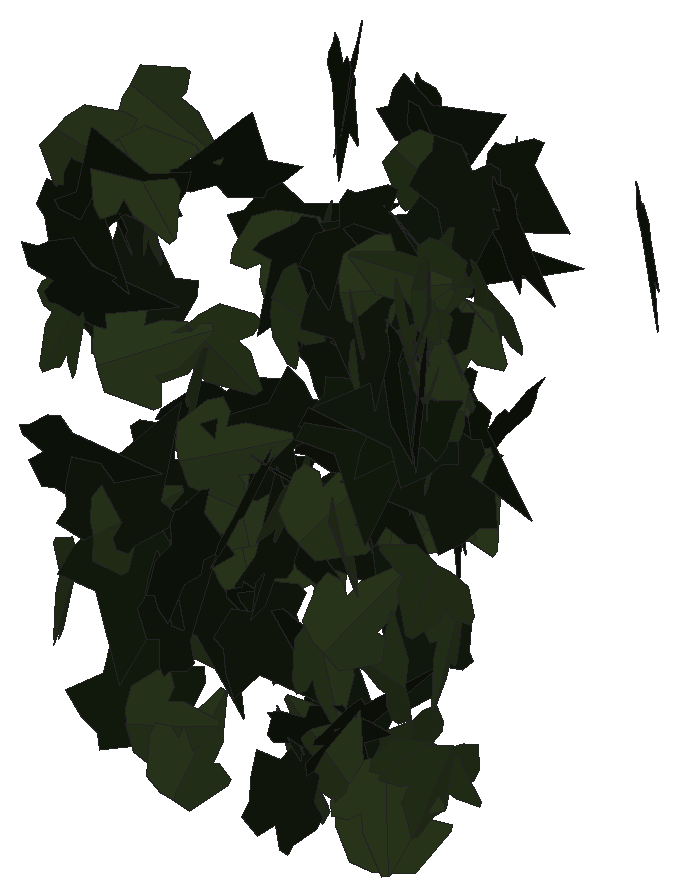
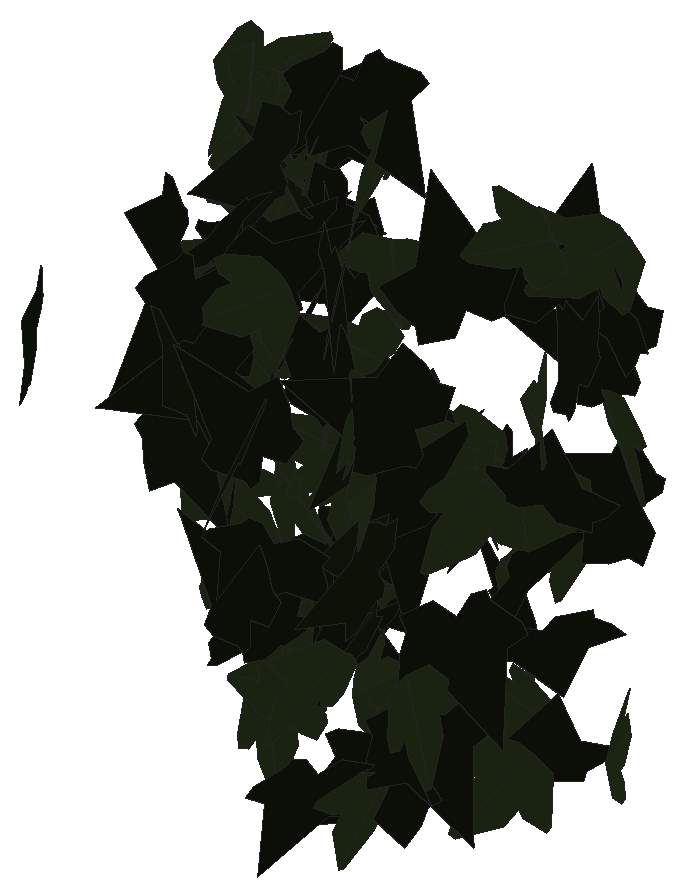
# SketchUp Ruby script. Lengths in inches.
U = 1.inch
M = Sketchup.active_model
def pt(a) = Geom::Point3d.new(a.map { |v| v * U })
def face(e, loops, mat)
  f = e.add_face(loops[0].map { |a| pt(a) })
  loops[1..].each { |l| e.add_face(l.map { |a| pt(a) }).erase! }
  f.material = f.back_material = mat if mat
  f
end
# faces: each face lists its corners as indices into pts; further lists are holes
def faces(e, pts, list, mat = nil) = list.each { |f| face(e, (f[0].is_a?(Array) ? f : [f]).map { |l| l.map { |i| pts[i] } }, mat) }
# xy, xz, yz: faces in a plane at the given z, y or x. An outline is a flat list of corners, or four numbers for a rectangle; further outlines are holes
def ring(l) = l.size == 4 ? [[l[0], l[1]], [l[2], l[1]], [l[2], l[3]], [l[0], l[3]]] : l.each_slice(2).to_a
def flat(e, list, mat, &to3) = list.each { |f| face(e, (f[0].is_a?(Array) ? f : [f]).map { |l| ring(l).map { |u, v| to3.(u, v) } }, mat) }
def xy(e, z, list, mat = nil) = flat(e, list, mat) { |x, y| [x, y, z] }
def xz(e, y, list, mat = nil) = flat(e, list, mat) { |x, z| [x, y, z] }
def yz(e, x, list, mat = nil) = flat(e, list, mat) { |y, z| [x, y, z] }
def lines(e, pts, list) = list.each { |a, b| e.add_line(pt(pts[a]), pt(pts[b])) }
# prism: a flat outline (further loops are holes) pulled along v
def prism(e, loops, v, mat = nil)
  f = face(e, loops, mat); d = Geom::Vector3d.new(v.map { |x| x * U })
  f.pushpull(f.normal.samedirection?(d) ? d.length : -d.length)
end
def box(e, o, s, mat = nil) = prism(e, [[o, [o[0] + s[0], o[1], o[2]], [o[0] + s[0], o[1] + s[1], o[2]], [o[0], o[1] + s[1], o[2]]]], [0, 0, s[2]], mat)
def at(x, y, z, deg = 0) = Geom::Transformation.translation(pt([x, y, z])) * Geom::Transformation.rotation(ORIGIN, Z_AXIS, deg.degrees)
def axes(o, x, y, z) = Geom::Transformation.new([*x, 0, *y, 0, *z, 0, *pt(o).to_a, 1])
def part(name) = M.definitions.add(name)
# library, detail: a bought-in or finely detailed component or shape, given as its bounding box
def library(name, o, s) = part(name).tap { |d| box(d.entities, o, s) }
def detail(e, o, s) = box(e.add_group.entities, o, s)
def put(e, d, t, mat = nil) = e.add_instance(d, t).tap { |i| i.material = mat if mat }
def group(e, t, mat = nil) = e.add_group.tap { |g| g.transformation = t; g.material = mat if mat }.entities
root = M.entities
M.materials.add("efeu1").color = [18, 25, 13]
M.materials.add("efeu2").color = [43, 57, 29]
c1 = part("ivyleaf_10")
p = [[0,0.5,-0.03],[-0.0625,2.02,-0.43],[-0.19,2.01,-0.46],[-0.54,1.05,-0.29],[-0.52,0.625,-0.18],[-0.83,0.76,-0.28],
  [-1.16,0.64,-0.33],[-1.15,0.33,-0.24],[-0.77,-0.39,0.02],[-0.3,-0.51,0.16],[0.04,-0.48,0.23],[-0.02,2.01,-0.4375],
  [-0.06,2.01,-0.43],[0.04,-0.49,0.23],[0.67,-0.49,0.14],[1.38,0.36,-0.2],[1.375,0.51,-0.24],[0.81,0.65,-0.19],
  [0.62,0.59,-0.15],[0.6,1.09,-0.28],[0.5,1.23,-0.31]]
faces(c1.entities,p,[[0,1,2,3,4,5,6,7,8,9,10],[11,12,0,13,14,15,16,17,18,19,20]],"efeu2")
c2 = part("ivyleaf_9")
p = [[1.54,2.16,1.25],[1.36,2.04,1.19],[-0.21,0.99,0.68],[-0.71,1.11,0.82],[-0.85,0.86,0.67],[-0.8,0.17,0.21],
  [-0.9,-0.01,0.1],[-0.67,-0.16,-0.02],[-0.08,-0.08,-0.05],[-0.03,-0.6,-0.4],[0.65,-0.88,-0.66],[0.83,-0.6,-0.49],
  [1.29,-0.42,-0.43],[1.8125,-0.07,-0.26],[1.21,0.44,0.15]]
faces(c2.entities,p,[[0,1,2,3,4,5,6,7,8,9,10,11,12,13,14]],"efeu1")
put(root,c1,axes([40.76,222.9,207.83],[0.02741,-0.09266,0.49057],[0.33181,-0.36372,-0.08723],[0.37303,0.33034,0.04155]))
put(root,c1,axes([41.28,222.25,211.54],[0.37477,-0.26819,-0.19397],[-0.14449,0.13106,-0.46038],[0.29778,0.40112,0.02073]))
put(root,c2,axes([41.35,223.39,210.93],[-0.48337,-0.04307,0.12042],[0.12298,-0.02733,0.48387],[-0.0351,0.49739,0.03702]))
put(root,c2,axes([40.98,223.26,212.49],[0.07585,-0.18054,0.46006],[0.17026,-0.42741,-0.1958],[0.46396,0.18636,-0.00336]))
put(root,c1,axes([41.03,223.82,212.2],[0.05825,-0.10838,0.48462],[0.43552,-0.22329,-0.10228],[0.2386,0.43404,0.06839]))
put(root,c1,axes([41.28,222.4,213.59],[-0.28359,-0.11302,-0.39599],[0.37792,0.11956,-0.30477],[0.16358,-0.47216,0.01761]))
put(root,c2,axes([41.17,222.34,212.94],[0.02257,-0.11058,-0.4871],[0.48167,0.13391,-0.00808],[0.13224,-0.46887,0.11257]))
put(root,c2,axes([41.74,224.34,209.75],[0.06056,0.38676,-0.31104],[-0.04519,-0.30775,-0.39147],[-0.49426,0.07553,-0.00232]))
put(root,c1,axes([41.7,225.14,209.18],[-0.00925,-0.49976,0.01246],[-0.00029,-0.01246,-0.49984],[0.49991,-0.00925,-0.00006]))
put(root,c1,axes([41.41,222.97,210.72],[0.15505,0.00567,-0.47532],[0.41334,0.24531,0.13776],[0.23476,-0.43565,0.07138]))
put(root,c2,axes([41.875,224.76,208.66],[0.05441,0.36351,-0.33897],[-0.03108,-0.33784,-0.36728],[-0.49606,0.06104,-0.01417]))
put(root,c2,axes([41.39,221.94,212.08],[0.25716,-0.07512,0.42216],[0.40897,-0.10498,-0.26781],[0.12888,0.48305,0.00745]))
put(root,c2,axes([41.83,222.51,212.86],[0.36961,0.10063,0.32135],[-0.30891,-0.08859,0.38305],[0.13403,-0.48169,-0.00332]))
put(root,c1,axes([41.72,223.42,207.56],[-0.40027,-0.11165,-0.27806],[0.26339,0.09014,-0.41533],[0.14287,-0.47897,-0.01335]))
put(root,c2,axes([41.45,221.69,210.11],[0.30415,0.13581,-0.37289],[0.30908,0.21361,0.32991],[0.24892,-0.43119,0.04599]))
put(root,c1,axes([41.66,223.11,213.86],[0.19523,0.07178,0.45468],[0.41972,0.17503,-0.20785],[-0.189,0.46283,0.00808]))
put(root,c2,axes([42,222.56,208.75],[-0.22161,-0.43487,-0.10852],[0.05116,0.09573,-0.48808],[0.44528,-0.22743,0.00207]))
put(root,c1,axes([41.98,223.64,210.875],[-0.29908,-0.28039,-0.28624],[0.23111,0.17107,-0.40905],[0.32732,-0.37698,0.02727]))
put(root,c2,axes([42.05,223.03,209.62],[0.10036,-0.21623,-0.43951],[0.23352,-0.37326,0.23696],[-0.43058,-0.25283,0.02607]))
put(root,c1,axes([42.02,224.22,208.68],[0.26022,0.41841,0.08496],[0.04478,0.0722,-0.49273],[-0.4246,0.26404,0.0001]))
put(root,c2,axes([42.31,222.32,206.94],[-0.43099,-0.20081,0.15466],[0.13908,0.06769,0.47547],[-0.2119,0.45287,-0.00249]))
put(root,c1,axes([41.99,222.41,213.55],[0.25807,0.36228,0.22837],[0.12907,0.18844,-0.44478],[-0.40834,0.28852,0.00375]))
put(root,c1,axes([42.16,225.2,207.94],[0.1165,0.45741,0.16492],[0.04885,0.15772,-0.47195],[-0.48378,0.12608,-0.00794]))
put(root,c2,axes([42.24,221.77,209.52],[-0.18502,-0.09603,0.45447],[0.38791,0.23717,0.20803],[-0.25553,0.42957,-0.01326]))
put(root,c1,axes([42.23,221.75,209.48],[0.02962,-0.0014,-0.49912],[0.19981,0.45822,0.01058],[0.45738,-0.20008,0.0277]))
put(root,c2,axes([42.08,225.0625,208.17],[-0.03362,-0.03078,-0.49792],[0.28186,0.41059,-0.04442],[0.41161,-0.28367,-0.01025]))
put(root,c1,axes([42.27,223.23,210.73],[0.26387,-0.34772,0.24385],[0.17033,-0.17634,-0.43576],[0.38905,0.31304,0.02539]))
put(root,c1,axes([42.6875,222.3,208.86],[-0.09901,0.15616,0.46455],[-0.30869,0.34824,-0.18285],[-0.38067,-0.32302,0.02745]))
put(root,c1,axes([42.43,225.71,209.56],[0.07082,0.37289,0.32548],[0.06458,0.31903,-0.37954],[-0.49073,0.09579,-0.00297]))
put(root,c2,axes([42.38,223.44,212.99],[0.42508,0.23101,0.12626],[-0.11086,-0.06042,0.4838],[0.23878,-0.4393,-0.00015]))
put(root,c2,axes([42.47,225.83,208.26],[-0.03598,-0.33878,-0.36597],[0.02404,0.36531,-0.34054],[0.49812,-0.0421,-0.01]))
put(root,c2,axes([42.45,224.86,210.32],[0.40943,-0.2849,0.03464],[0.0283,-0.01997,-0.4988],[0.2856,0.41041,-0.00023]))
put(root,c1,axes([42.61,223.61,208.21],[0.35489,0.33355,0.11314],[0.08399,0.07583,-0.48703],[-0.34205,0.36468,-0.0022]))
put(root,c2,axes([42.41,224.32,211.88],[0.1226,-0.00205,0.48473],[0.47854,0.08022,-0.12069],[-0.07728,0.49352,0.02163]))
put(root,c2,axes([43.11,224.77,213.85],[-0.07449,0.02563,-0.49375],[-0.45506,0.19169,0.0786],[0.19332,0.46109,-0.00523]))
put(root,c1,axes([43.06,224.34,211.77],[-0.01478,0.0005,0.49978],[-0.30463,0.39637,-0.0094],[-0.39621,-0.30477,-0.01141]))
put(root,c2,axes([42.87,226.3,212.77],[0.33533,-0.22409,-0.29552],[-0.24715,0.16203,-0.40331],[0.27653,0.41657,-0.0021]))
put(root,c2,axes([42.82,221.93,208.26],[-0.15694,0.25554,0.40009],[0.21378,-0.3382,0.29986],[0.42388,0.26518,-0.0031]))
put(root,c2,axes([42.78,225.05,213.78],[0.07054,-0.03168,-0.49399],[0.44675,-0.21079,0.07731],[-0.21316,-0.45229,-0.00143]))
put(root,c1,axes([42.69,221.84,207.18],[0.13058,-0.05009,-0.48004],[0.46569,-0.1176,0.13895],[-0.12682,-0.48339,0.01594]))
put(root,c2,axes([42.9,222.48,208.59],[0.22977,-0.44402,0.00716],[0.00328,-0.00637,-0.49995],[0.44407,0.22979,-0.00001]))
put(root,c2,axes([42.85,226.33,212.32],[-0.02801,-0.02484,0.4986],[0.42592,-0.26167,0.01088],[0.2604,0.42534,0.03582]))
put(root,c1,axes([43.08,224.23,210.93],[-0.22852,0.25827,-0.36204],[0.21497,-0.29218,-0.34412],[-0.38932,-0.31293,0.0225]))
put(root,c2,axes([43.39,223.38,210.125],[-0.0082,-0.00676,0.49989],[-0.32379,-0.38085,-0.01046],[0.38091,-0.32389,0.00186]))
put(root,c2,axes([43.42,221.375,209.8],[0.0244,0.02408,-0.49882],[-0.32328,0.38142,0.0026],[0.38065,0.32239,0.03419]))
put(root,c1,axes([43.29,221.65,206.82],[0.144,0.33645,-0.34068],[0.132,0.31407,0.36597],[0.46026,-0.19534,0.00163]))
put(root,c1,axes([43.41,225.15,208.43],[0.49526,0.04834,0.0488],[-0.05174,0.02891,0.49647],[0.04518,-0.49682,0.03363]))
put(root,c1,axes([43.1,222.28,210.42],[0.14237,0.02604,-0.47859],[0.46794,0.10049,0.14467],[0.10372,-0.4891,0.00425]))
put(root,c1,axes([43.66,223.01,212.96],[0.45686,0.20315,0.00174],[-0.0005,0.00541,-0.49997],[-0.20316,0.45684,0.00514]))
put(root,c2,axes([44.13,221.61,210.3],[-0.26634,0.24028,-0.34832],[-0.26596,0.22507,0.35862],[0.32913,0.37631,0.00791]))
put(root,c2,axes([43.75,224.97,210.24],[-0.15493,-0.23915,-0.41086],[0.25552,0.3225,-0.28408],[0.40088,-0.29799,0.02229]))
put(root,c1,axes([43.95,224.82,213.17],[-0.29925,0.00512,-0.40053],[0.39815,-0.05095,-0.29813],[-0.04387,-0.49737,0.02641]))
put(root,c2,axes([44.5625,221.66,209.74],[-0.37699,0.19823,-0.26189],[-0.24338,0.09913,0.42537],[0.22057,0.44819,0.02175]))
put(root,c2,axes([44.4375,221.76,209.16],[0.32902,0.14289,-0.34832],[-0.33469,-0.10083,-0.35751],[-0.17241,0.46842,0.02929]))
put(root,c2,axes([43.98,225.11,209.4],[0.03322,-0.01939,0.49852],[0.34242,-0.36247,-0.03692],[0.36283,0.34386,-0.0108]))
put(root,c2,axes([44.04,222.87,209.33],[0.31527,-0.36986,0.1175],[0.07693,-0.08882,-0.486],[0.38037,0.32452,0.0009]))
put(root,c1,axes([44.43,222.15,210.53],[0.09614,-0.48036,-0.10008],[-0.01476,0.0991,-0.48986],[0.49045,0.09714,0.00487]))
put(root,c2,axes([44.25,222.22,210.58],[0.48313,0.07785,-0.10261],[-0.11934,0.12065,-0.47032],[-0.04847,0.47894,0.13516]))
put(root,c1,axes([44.73,222.14,206.92],[-0.22144,0.20873,-0.39674],[-0.31456,0.24292,0.30338],[0.3194,0.38396,0.02373]))
put(root,c2,axes([44.62,225.44,212.3125],[0.00411,0.18855,0.46307],[-0.05767,0.46017,-0.18686],[-0.49665,-0.05188,0.02553]))
put(root,c2,axes([44.43,221.5,209.25],[0.14234,-0.2585,-0.40363],[-0.17096,0.36598,-0.29467],[0.44778,0.2219,0.0158]))
put(root,c2,axes([44.81,224.09,212.58],[-0.05854,-0.0085,0.49649],[-0.44355,-0.22387,-0.05613],[0.22325,-0.447,0.01867]))
put(root,c2,axes([44.4,224.89,212.09],[0.3272,0.1568,0.34403],[0.31355,0.14167,-0.36279],[-0.21125,0.45315,-0.00561]))
put(root,c1,axes([44.92,221.75,208.84],[0.1386,-0.0728,0.47486],[-0.33751,0.33695,0.15016],[-0.34187,-0.36216,0.04426]))
put(root,c2,axes([44.68,221.58,206.8125],[-0.31283,0.30419,0.24414],[0.17557,-0.16965,0.43634],[0.3483,0.35873,-0.00068]))
put(root,c2,axes([44.88,222.44,207.36],[-0.23483,-0.30328,0.32074],[0.19341,0.25588,0.38356],[-0.39679,0.30422,-0.00286]))
put(root,c2,axes([44.76,225.07,213.11],[0.03229,-0.10468,-0.48785],[-0.16592,0.4588,-0.10943],[0.47056,0.16896,-0.0051]))
put(root,c1,axes([44.95,221.4,213.26],[-0.09326,0.31932,0.37328],[-0.12662,0.35149,-0.3323],[-0.47463,-0.15651,0.0153]))
put(root,c2,axes([44.6,222.61,207.52],[0.20965,-0.38053,0.24746],[0.13275,-0.20927,-0.43426],[0.43408,0.24779,0.01328]))
put(root,c2,axes([45.125,223.7,207.97],[-0.2782,-0.4005,0.11049],[0.06279,0.09091,0.48764],[-0.41069,0.2852,-0.00029]))
put(root,c2,axes([45.13,221.8125,213.96],[0.0545,0.28843,-0.40477],[-0.06071,-0.40029,-0.2934],[-0.4933,0.08113,-0.00861]))
put(root,c1,axes([45.05,223.36,207.2],[-0.08166,-0.49133,-0.0439],[0.0097,0.04288,-0.49806],[0.49319,-0.0822,0.00253]))
put(root,c2,axes([44.89,224.6,213.42],[-0.0025,-0.48845,0.10681],[-0.01151,-0.10673,-0.48834],[0.49986,-0.0049,-0.01071]))
put(root,c2,axes([44.73,222.8,210.83],[-0.027,0.02642,0.49857],[0.35336,-0.35172,0.03777],[0.35271,0.35439,0.00033]))
put(root,c2,axes([45.01,221.7,208.08],[0.41121,0.27936,-0.0535],[-0.04636,-0.02696,-0.49712],[-0.28063,0.4138,0.00373]))
put(root,c2,axes([44.82,224.39,209.78],[0.05875,-0.03449,-0.49534],[0.46618,-0.16789,0.06699],[-0.17094,-0.46971,0.01243]))
put(root,c1,axes([45.43,221.68,207.69],[0.2341,0.02823,0.44091],[-0.44181,0.01285,0.23375],[0.00186,-0.49904,0.03096]))
put(root,c1,axes([45.32,223.92,209.99],[0.39722,0.09566,-0.28821],[-0.27962,-0.06989,-0.40857],[-0.11845,0.48576,-0.00203]))
put(root,c1,axes([45.24,221.625,209.18],[0.05083,0.49572,0.04096],[0.00282,0.04089,-0.49832],[-0.4974,0.05089,0.00136]))
put(root,c2,axes([45.28,221.94,214.08],[0.05553,-0.08502,-0.48958],[-0.14629,0.468,-0.09787],[0.47489,0.15411,0.0271]))
put(root,c1,axes([45.47,221.64,210.53],[-0.30311,0.32639,0.22715],[-0.1494,0.17122,-0.44538],[-0.36852,-0.33787,-0.00627]))
put(root,c1,axes([45.17,221.59,210.59],[0.21536,0.20763,-0.40064],[0.28912,0.27735,0.29915],[0.34646,-0.36051,-0.0006]))
put(root,c2,axes([45.32,221.66,207.95],[-0.0509,0.42894,-0.25184],[-0.02821,0.25026,0.43194],[0.4966,0.05818,-0.00128]))
put(root,c2,axes([45.59,224.35,210.84],[-0.22462,0.37913,-0.23624],[0.11095,-0.20879,-0.44057],[-0.43271,-0.25034,0.00967]))
put(root,c2,axes([45.65,223.125,212.09],[-0.05829,-0.04688,0.49437],[-0.37409,-0.32322,-0.07476],[0.32659,-0.37859,0.00261]))
put(root,c1,axes([45.52,223.55,212.33],[0.41516,0.2177,-0.17392],[-0.15289,-0.08294,-0.46877],[-0.23295,0.44241,-0.0023]))
put(root,c2,axes([45.13,222.05,212.625],[0.01084,-0.10676,-0.48835],[0.42871,0.25319,-0.04584],[0.25708,-0.41773,0.09703]))
put(root,c1,axes([45.71,223.92,212.51],[-0.41105,0.13441,0.25095],[-0.2359,0.08589,-0.4324],[-0.15935,-0.47387,-0.0072]))
put(root,c2,axes([45.2,223.1,213.54],[0.39686,-0.26695,0.14574],[0.12703,-0.07222,-0.47817],[0.27635,0.41656,0.0105]))
put(root,c1,axes([45.55,221.89,213.26],[-0.21677,0.45047,-0.00939],[0.00231,-0.00931,-0.49991],[-0.45056,-0.21678,0.00196]))
put(root,c1,axes([45.53,223.33,212.49],[0.1366,-0.36781,0.30994],[0.11889,-0.28638,-0.39224],[0.46605,0.18085,0.00922]))
put(root,c2,axes([45.32,221.55,211.71],[0.37429,0.09864,0.31651],[0.30391,0.08867,-0.38701],[-0.13248,0.48209,0.00642]))
put(root,c1,axes([45.46,221.64,209.33],[0.20072,0.22011,-0.40158],[0.27059,0.29673,0.29788],[0.36945,-0.33691,0]))
put(root,c2,axes([45.57,222.04,211.22],[0.30368,-0.23757,-0.31834],[-0.23277,0.21827,-0.38494],[0.32186,0.382,0.02197]))
put(root,c2,axes([45.73,223.07,211.46],[0.10103,-0.10882,-0.47744],[-0.32415,0.35054,-0.14849],[0.36704,0.33953,0.00028]))
put(root,c1,axes([46.07,221.9,208.85],[-0.05248,0.04571,0.49513],[-0.48638,0.09874,-0.06067],[-0.10333,-0.48802,0.0341]))
put(root,c1,axes([45.71,221.84,212.8],[-0.08119,0.44324,0.21667],[-0.03826,0.21327,-0.45062],[-0.49188,-0.08975,-0.00072]))
put(root,c2,axes([45.6,221.83,213.51],[-0.30771,-0.1775,-0.35186],[0.3036,0.17787,-0.35523],[0.25128,-0.43227,-0.00169]))
put(root,c2,axes([45.38,223.65,211.08],[-0.00575,0.00203,-0.49996],[0.46014,0.19558,-0.0045],[0.19554,-0.46016,-0.00412]))
put(root,c2,axes([45.4,224.51,213.16],[0.13466,-0.05504,-0.47837],[0.48152,0.01696,0.1336],[0.00152,-0.49667,0.05758]))
put(root,c2,axes([45.74,221.92,212.05],[-0.20079,-0.43889,-0.13061],[0.07246,0.11037,-0.48225],[0.45214,-0.21259,0.01928]))
put(root,c2,axes([45.83,222.02,212.74],[-0.29619,0.40152,0.03249],[0.01753,-0.02744,0.49894],[0.40245,0.2967,0.00218]))
put(root,c1,axes([45.83,222.01,206.68],[0.31985,0.37533,-0.08258],[0.04847,0.06718,0.49309],[0.38124,-0.32344,0.00659]))
put(root,c1,axes([45.82,221.95,207.49],[0.45954,0.18285,0.07341],[0.06742,0.0291,-0.49458],[-0.18514,0.46446,0.00208]))
put(root,c1,axes([45.67,221.8125,213.55],[0.12529,-0.04142,-0.48227],[0.48231,0.05288,0.12076],[0.041,-0.49547,0.0532]))
put(root,c2,axes([45.79,221.85,212.93],[-0.07437,-0.05298,-0.49159],[0.49226,0.03866,-0.07864],[0.04634,-0.49568,0.04641]))
put(root,c1,axes([46.1875,221.9375,213.02],[-0.27307,0.37065,0.19507],[-0.11389,0.15839,-0.46037],[-0.40306,-0.29586,-0.00208]))
put(root,c1,axes([46.19,222.17,212.67],[0.46313,0.12647,-0.13969],[-0.1747,0.14927,-0.44407],[-0.07062,0.46013,0.18245]))
put(root,c1,axes([46.38,222.13,213.71],[-0.16414,-0.12972,-0.45413],[-0.36881,-0.26511,0.20903],[-0.29502,0.4036,-0.00865]))
put(root,c1,axes([46.09,222.76,209.22],[0.38689,-0.30676,0.07885],[0.06365,-0.04664,-0.49373],[0.31027,0.39208,0.00296]))
put(root,c1,axes([45.83,222.7,210.74],[0.3217,-0.063,-0.37754],[0.37502,-0.0468,0.32736],[-0.07658,-0.4938,0.01714]))
put(root,c1,axes([46.43,221.98,212.37],[0.00778,0.14514,0.47841],[-0.40727,0.27933,-0.07812],[-0.28994,-0.38847,0.12257]))
put(root,c1,axes([46.17,221.93,213.58],[-0.18262,0.44532,0.13541],[-0.05216,0.12496,-0.48131],[-0.46252,-0.18992,0.00081]))
put(root,c1,axes([46.27,222.11,207.83],[0.47027,0.13736,-0.09989],[-0.14964,0.196,-0.43496],[-0.08033,0.43899,0.22546]))
put(root,c1,axes([46.26,222.22,211.76],[0.33995,-0.3628,-0.05299],[-0.03631,0.0386,-0.49718],[0.36485,0.34188,-0.0001]))
put(root,c2,axes([46.4,222.07,212.19],[-0.00418,-0.39264,-0.30955],[-0.00589,-0.3095,0.39265],[-0.49995,0.00693,-0.00204]))
put(root,c2,axes([46.46,222.01,212.49],[-0.4991,0.01126,-0.02777],[0.02777,-0.00024,-0.49923],[-0.01126,-0.49987,-0.00039]))
put(root,c2,axes([46,226.17,212.61],[0.05972,-0.01061,-0.49631],[0.47416,-0.1468,0.06019],[-0.147,-0.47785,-0.00747]))
put(root,c1,axes([46.66,222,212.41],[0.04144,0.04655,0.4961],[-0.48562,-0.10771,0.05068],[0.11159,-0.48604,0.03629]))
put(root,c1,axes([46.375,222.01,213.68],[-0.04802,0.17732,0.46503],[-0.17401,0.43172,-0.18259],[-0.46628,-0.17938,0.02025]))
put(root,c1,axes([46.52,221.93,210.27],[-0.44379,-0.05856,0.22277],[-0.21736,-0.05351,-0.44709],[0.0762,-0.49367,0.02203]))
put(root,c1,axes([46.55,221.74,213.61],[0.068,-0.24011,-0.43327],[-0.13396,0.41212,-0.24941],[0.4769,0.15,-0.00829]))
put(root,c1,axes([46.52,222.1,207.93],[-0.16554,-0.45439,0.12699],[-0.0527,-0.11594,-0.48351],[0.46885,-0.17347,-0.00951]))
put(root,c2,axes([46.65,221.53,212.68],[-0.00846,0.06264,-0.49599],[-0.45432,0.20604,0.03377],[0.20862,0.45125,0.05343]))
put(root,c2,axes([46.8125,222.12,211.51],[-0.12944,-0.13135,-0.46475],[-0.3281,-0.32916,0.18441],[-0.3544,0.3527,-0.00098]))
put(root,c1,axes([46.11,222.19,212.91],[0.22543,0.00747,0.44623],[0.44627,0.00165,-0.22548],[-0.00484,0.49994,-0.00592]))
